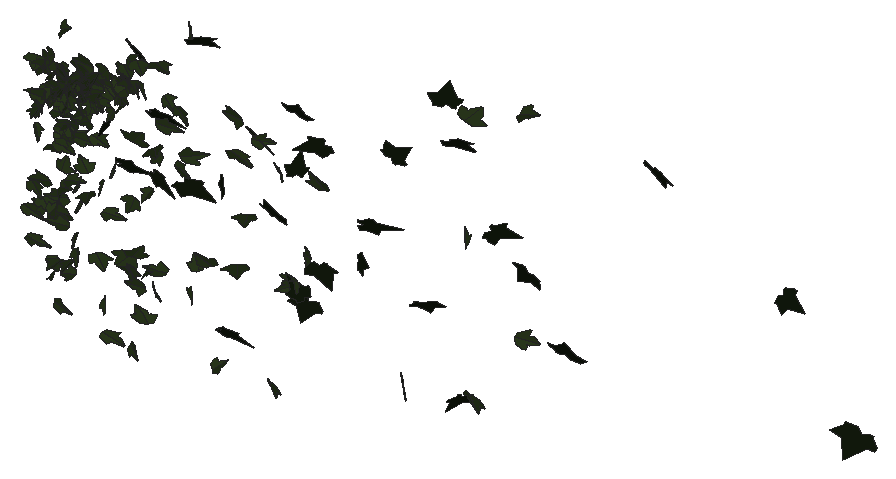
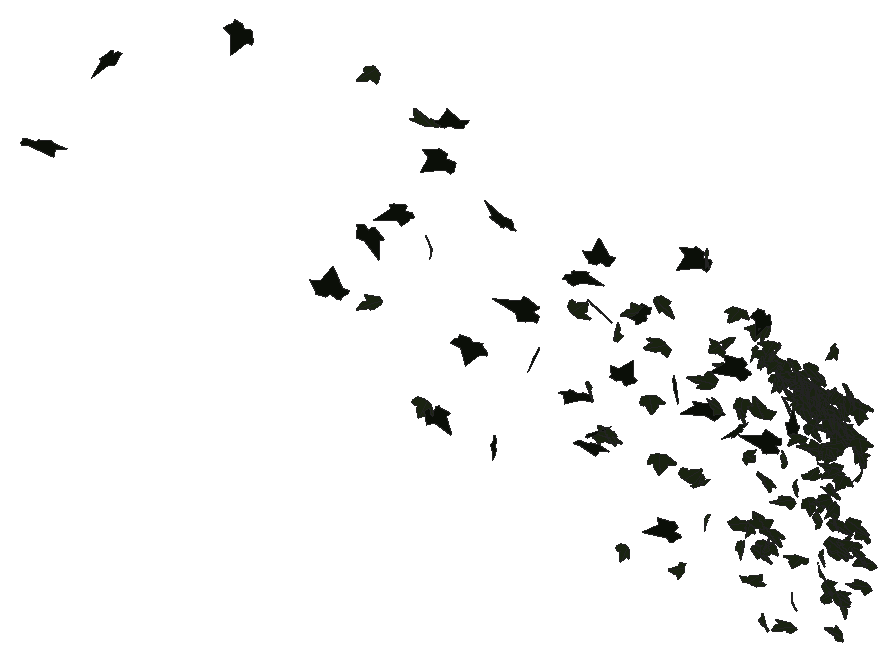
# SketchUp Ruby script. Lengths in millimetres.
U = 1.mm
M = Sketchup.active_model
def pt(a) = Geom::Point3d.new(a.map { |v| v * U })
def face(e, loops, mat)
  f = e.add_face(loops[0].map { |a| pt(a) })
  loops[1..].each { |l| e.add_face(l.map { |a| pt(a) }).erase! }
  f.material = f.back_material = mat if mat
  f
end
# faces: each face lists its corners as indices into pts; further lists are holes
def faces(e, pts, list, mat = nil) = list.each { |f| face(e, (f[0].is_a?(Array) ? f : [f]).map { |l| l.map { |i| pts[i] } }, mat) }
# xy, xz, yz: faces in a plane at the given z, y or x. An outline is a flat list of corners, or four numbers for a rectangle; further outlines are holes
def ring(l) = l.size == 4 ? [[l[0], l[1]], [l[2], l[1]], [l[2], l[3]], [l[0], l[3]]] : l.each_slice(2).to_a
def flat(e, list, mat, &to3) = list.each { |f| face(e, (f[0].is_a?(Array) ? f : [f]).map { |l| ring(l).map { |u, v| to3.(u, v) } }, mat) }
def xy(e, z, list, mat = nil) = flat(e, list, mat) { |x, y| [x, y, z] }
def xz(e, y, list, mat = nil) = flat(e, list, mat) { |x, z| [x, y, z] }
def yz(e, x, list, mat = nil) = flat(e, list, mat) { |y, z| [x, y, z] }
def lines(e, pts, list) = list.each { |a, b| e.add_line(pt(pts[a]), pt(pts[b])) }
# prism: a flat outline (further loops are holes) pulled along v
def prism(e, loops, v, mat = nil)
  f = face(e, loops, mat); d = Geom::Vector3d.new(v.map { |x| x * U })
  f.pushpull(f.normal.samedirection?(d) ? d.length : -d.length)
end
def box(e, o, s, mat = nil) = prism(e, [[o, [o[0] + s[0], o[1], o[2]], [o[0] + s[0], o[1] + s[1], o[2]], [o[0], o[1] + s[1], o[2]]]], [0, 0, s[2]], mat)
def at(x, y, z, deg = 0) = Geom::Transformation.translation(pt([x, y, z])) * Geom::Transformation.rotation(ORIGIN, Z_AXIS, deg.degrees)
def axes(o, x, y, z) = Geom::Transformation.new([*x, 0, *y, 0, *z, 0, *pt(o).to_a, 1])
def part(name) = M.definitions.add(name)
# library, detail: a bought-in or finely detailed component or shape, given as its bounding box
def library(name, o, s) = part(name).tap { |d| box(d.entities, o, s) }
def detail(e, o, s) = box(e.add_group.entities, o, s)
def put(e, d, t, mat = nil) = e.add_instance(d, t).tap { |i| i.material = mat if mat }
def group(e, t, mat = nil) = e.add_group.tap { |g| g.transformation = t; g.material = mat if mat }.entities
root = M.entities
M.materials.add("efeu1").color = [18, 25, 13]
M.materials.add("efeu2").color = [43, 57, 29]
c1 = part("ivyleaf_10")
p = [[0,12.8,-0.8],[-1.5,51.3,-10.9],[-4.9,51,-11.6],[-13.6,26.5,-7.3],[-13.2,15.9,-4.6],[-21.1,19.3,-7.2],
  [-29.5,16.3,-8.3],[-29.2,8.3,-6.2],[-19.7,-9.8,0.5],[-7.6,-13,4],[1,-12.2,5.8],[-0.4,51.1,-11.1],
  [-1.5,51.1,-10.9],[1,-12.4,5.9],[16.9,-12.4,3.5],[35.1,9.1,-5.1],[35,12.9,-6.1],[20.5,16.4,-4.9],
  [15.8,15,-3.8],[15.3,27.6,-7.1],[12.8,31.3,-7.8]]
faces(c1.entities,p,[[0,1,2,3,4,5,6,7,8,9,10],[11,12,0,13,14,15,16,17,18,19,20]],"efeu2")
c2 = part("ivyleaf_9")
p = [[39.1,54.8,31.7],[34.5,51.8,30.2],[-5.3,25.2,17.3],[-17.9,28.3,20.9],[-21.6,21.7,17],[-20.2,4.3,5.3],
  [-22.9,-0.3,2.5],[-17.1,-4,-0.6],[-2,-2.1,-1.2],[-0.7,-15.4,-10.1],[16.6,-22.3,-16.7],[21.1,-15.1,-12.5],
  [32.7,-10.7,-11],[46.1,-1.8,-6.6],[30.8,11.2,3.8]]
faces(c2.entities,p,[[0,1,2,3,4,5,6,7,8,9,10,11,12,13,14]],"efeu1")
put(root,c1,axes([1688.4,1054.2,385.2],[0.66637,0.14014,0.53567],[0.92513,0.22568,-0.37677],[-0.5046,0.59883,0.01663]))
put(root,c1,axes([1715.8,1060.3,753.9],[-0.9466,-0.39098,0.07189],[-0.06525,-0.07252,-0.63165],[0.75376,-0.49728,0.0356]))
put(root,c1,axes([1722.4,1052.4,705.3],[-0.276,-0.61082,0.15015],[-0.05742,-0.14715,-0.62778],[1.19573,-0.14805,0.00451]))
put(root,c1,axes([1727,1052.4,841.1],[-1.14001,0.22774,0.16973],[-0.33916,0.00715,-0.63849],[-0.42094,-0.62254,0.05476]))
put(root,c1,axes([1733.3,1055.6,406],[0.74106,-0.32591,-0.41907],[-0.6286,0.25817,-0.50765],[0.79103,0.51047,-0.01081]))
put(root,c1,axes([1721.7,1052.9,706.2],[0.74402,-0.51019,-0.0648],[0.0973,0.11954,-0.63278],[0.97394,0.3778,0.11272]))
put(root,c1,axes([1747.1,1057.4,489.3],[-0.51143,-0.04017,0.6118],[-1.13991,-0.12561,-0.27132],[0.24947,-0.6563,0.01448]))
put(root,c1,axes([1721.3,1049,863.4],[1.25976,0.08591,-0.01452],[-0.02826,0.00162,-0.66746],[-0.1634,0.66207,0.00352]))
put(root,c1,axes([1721,1050.8,649.2],[-0.04462,0.68269,-0.2239],[0.02754,-0.22352,-0.68306],[-1.36711,-0.02678,-0.00645]))
put(root,c1,axes([1709.9,1051.4,464.6],[0.90696,-0.15382,0.43059],[0.81416,-0.06963,-0.49831],[0.3073,0.63848,0.04939]))
put(root,c1,axes([1708.6,1045.4,301.5],[-0.4079,-0.06195,-0.61418],[1.1745,-0.03684,-0.21164],[-0.02771,-0.64945,0.07059]))
put(root,c1,axes([1742.5,1040.1,717.7],[0.01577,0.21516,-0.621],[-0.32952,0.59982,0.20552],[1.20663,0.161,0.06424]))
put(root,c1,axes([1755.7,1045.9,879.3],[0.32299,-0.47142,-0.46343],[-0.27462,0.44051,-0.50094],[1.2278,0.22254,0.00987]))
put(root,c1,axes([1723.1,1048.2,748],[0.12374,-0.0032,0.76231],[1.17016,0.45253,-0.05054],[-0.85772,0.6169,0.04103]))
put(root,c1,axes([1747.7,1052.8,758],[-0.52103,0.57291,-0.11289],[0.06869,-0.10785,-0.63481],[-1.1092,-0.27579,0.01372]))
put(root,c1,axes([1753.9,1052,750.8],[0.3947,-0.62861,-0.08831],[-0.02203,0.08915,-0.66172],[1.20791,0.20703,0.01679]))
put(root,c1,axes([1742.8,1055.4,426.1],[0.88803,0.42819,0.2143],[0.29282,0.14928,-0.63327],[-0.86298,0.49128,0.00564]))
put(root,c1,axes([1755,1048,863.6],[-1.09124,-0.35064,-0.07902],[0.18739,-0.01014,-0.66944],[0.65791,-0.5787,0.05961]))
put(root,c1,axes([1774.4,1049.3,777.5],[-0.54687,0.54467,0.20836],[-0.53322,0.07478,-0.58186],[-0.97339,-0.34697,0.20167]))
put(root,c1,axes([1774.2,1058.6,754.8],[-0.56025,-0.55661,0.109],[-0.02811,-0.11524,-0.62837],[1.07909,-0.29199,0.04022]))
put(root,c1,axes([1772.1,1059.5,774.4],[-0.28489,-0.41914,0.45869],[0.11153,-0.47923,-0.41879],[1.17728,-0.05603,0.15067]))
put(root,c1,axes([1778.9,1044.2,895.9],[0.48867,-0.47376,-0.42549],[-0.33643,0.38772,-0.53837],[1.1643,0.31088,0.02302]))
put(root,c1,axes([1775,1051.4,834],[-0.03031,-0.63857,-0.21042],[0.05202,0.20969,-0.63842],[1.27855,-0.02367,0.02099]))
put(root,c1,axes([1750.8,1057.4,778.3],[0.66661,0.03309,0.54247],[0.99021,0.16609,-0.34607],[-0.29891,0.62399,0.06335]))
put(root,c1,axes([1792.1,1056.1,398.3],[-1.02972,-0.15447,0.32085],[-0.55712,-0.13937,-0.56073],[0.3859,-0.61339,0.04661]))
put(root,c1,axes([1776.2,1058.6,775],[1.18689,-0.12873,-0.0014],[-0.00141,0.00332,-0.63677],[0.24502,0.62362,0.0031]))
put(root,c1,axes([1784.3,1047.1,222.2],[0.10096,-0.69928,-0.18249],[-0.01953,0.18224,-0.70128],[1.37531,0.05392,0.00344]))
put(root,c1,axes([1789.2,1057.7,251.6],[-0.40036,-0.48272,0.36837],[-0.23435,-0.34784,-0.52613],[1.13165,-0.24281,0.02137]))
put(root,c1,axes([1781.2,1051.9,612.5],[-0.70473,-0.48383,-0.30882],[0.34511,0.25008,-0.60922],[1.03646,-0.41224,-0.00713]))
put(root,c1,axes([1779.1,1040.1,411.1],[0.18254,0.28812,-0.61732],[0.37154,0.58564,0.30366],[1.24217,-0.21751,-0.00011]))
put(root,c1,axes([1798.2,1047.7,858.8],[-0.93446,0.33264,0.32838],[-0.53915,0.16705,-0.59279],[-0.70759,-0.56657,0.01801]))
put(root,c1,axes([1814,1059.2,407.7],[-0.56702,-0.02674,0.67681],[-1.27662,-0.091,-0.29887],[0.17897,-0.73386,0.0124]))
put(root,c1,axes([1792,1058.9,785.4],[-0.09638,-0.64206,-0.09498],[0.00722,0.09497,-0.64404],[1.23525,-0.05065,-0.00365]))
put(root,c1,axes([1766.2,1059.4,241.1],[0.2426,-0.08265,-0.6202],[1.15061,-0.14678,0.14381],[-0.30677,-0.61592,0.04895]))
put(root,c1,axes([1812.5,1050.2,462.3],[0.55085,-0.04814,-0.61462],[-1.14383,0.12923,-0.29315],[0.2614,0.66695,0.01244]))
put(root,c1,axes([1814.1,1052.4,375.5],[-0.00216,0.06306,0.64759],[-1.06342,-0.33192,0.03134],[0.63451,-0.55607,0.05473]))
put(root,c1,axes([1804.1,1057.8,795.5],[-0.30932,-0.626,0.08958],[-0.02902,-0.08858,-0.64671],[1.20318,-0.16307,0.00743]))
put(root,c1,axes([1800.8,1047.7,810],[-1.2279,-0.08263,-0.08152],[0.15996,-0.01502,-0.64995],[0.15236,-0.65013,0.02537]))
put(root,c1,axes([1804.7,1061.7,791.1],[0.06932,-0.63597,0.0421],[0.03119,-0.04122,-0.63686],[1.21263,0.03741,0.01397]))
put(root,c1,axes([1790,1051.7,721.8],[-0.35685,-0.20395,-0.57631],[0.92204,0.31807,-0.27018],[0.7096,-0.51586,0.06125]))
put(root,c1,axes([1806.8,1054.3,478.7],[0.39772,-0.63713,0.11459],[0.0925,-0.10464,-0.6704],[1.22857,0.21413,0.01338]))
put(root,c1,axes([1809.9,1047.5,792.2],[0.07675,-0.60534,-0.30444],[-0.00284,0.3049,-0.60645],[1.28957,0.0367,0.01678]))
put(root,c1,axes([1807.3,1056.1,819],[0.86009,-0.45158,-0.15955],[0.04049,0.23808,-0.61358],[0.91062,0.41594,0.17798]))
put(root,c1,axes([1794.8,1049.2,863],[1.1388,-0.14425,0.27817],[0.57836,0.12093,-0.59097],[0.14543,0.64868,0.17203]))
put(root,c1,axes([1806.5,1056.5,807.1],[0.78841,-0.50056,0.10032],[0.19872,-0.04339,-0.64765],[0.95107,0.42402,0.05216]))
put(root,c1,axes([1818.6,1062.7,780.6],[-0.60959,-0.53428,0.14995],[-0.00777,-0.17086,-0.61751],[1.0561,-0.30965,0.082]))
put(root,c1,axes([1794,1051.3,121.6],[0.06512,-0.00782,0.66223],[1.23192,-0.13988,-0.0351],[0.26664,0.64819,0.00042]))
put(root,c1,axes([1803.5,1049.7,624.5],[0.64809,0.33834,0.47524],[0.57678,0.3676,-0.47886],[-0.9487,0.45462,0.03352]))
put(root,c1,axes([1820.2,1061.9,798.4],[0.95344,0.35528,-0.1951],[-0.28637,-0.125,-0.614],[-0.71629,0.52288,-0.01422]))
put(root,c1,axes([1813.6,1050.9,552.8],[1.20898,-0.26037,-0.02043],[0.05955,0.02252,0.68574],[-0.49347,-0.63516,0.03269]))
put(root,c1,axes([1816.8,1053,753.2],[1.09075,0.28141,-0.0286],[-0.04777,-0.01377,-0.63848],[-0.53621,0.57366,-0.00129]))
put(root,c1,axes([1817.6,1046.7,868.5],[-0.34724,0.65594,0.01519],[0.02036,0.01874,-0.68067],[-1.24856,-0.18212,-0.01533]))
put(root,c1,axes([1800.1,1050.8,640.1],[0.35137,-0.03693,-0.66129],[1.11581,0.32849,0.14533],[0.58644,-0.6029,0.11969]))
put(root,c1,axes([1833.9,1055.2,695.9],[-0.89828,-0.30961,0.2979],[-0.447,-0.18464,-0.56402],[0.68473,-0.52671,0.02261]))
put(root,c1,axes([1824.3,1057.9,808.5],[1.15834,-0.1362,-0.15762],[-0.25909,0.10836,-0.61931],[0.30008,0.6193,0.0737]))
put(root,c1,axes([1822.1,1036,994.9],[-0.04137,-0.32316,-0.72112],[0.29892,0.70523,-0.32077],[1.47393,-0.1521,0.04481]))
put(root,c1,axes([1821.8,1034.8,505],[-0.13223,-0.44392,-0.63667],[0.44717,0.5972,-0.44204],[1.40788,-0.23137,0.0806]))
put(root,c1,axes([1832.6,1055.1,265.2],[-0.14744,-0.65397,0.2853],[-0.09712,-0.28116,-0.65834],[1.35444,-0.09135,-0.01615]))
put(root,c1,axes([1828.6,1042.7,754.3],[-0.0496,-0.38595,-0.51186],[0.0927,0.50961,-0.38673],[1.21654,-0.05457,0.0086]))
put(root,c1,axes([1812.7,1038.1,684.3],[0.30124,0.14682,0.65035],[0.53447,0.59156,-0.2019],[-1.15085,0.31316,0.07647]))
put(root,c1,axes([1831.9,1052.3,693.3],[-0.38434,-0.57345,-0.30825],[0.24766,0.28067,-0.6074],[1.21408,-0.23879,0.02632]))
put(root,c1,axes([1847.6,1041.2,680.7],[0.21327,0.00148,-0.71032],[-0.66242,0.62698,-0.0536],[1.17848,0.35216,0.09842]))
put(root,c1,axes([1833.3,1053.7,818.3],[-1.24449,0.00582,-0.06624],[0.12617,0.00603,-0.65389],[-0.00986,-0.65721,-0.00659]))
put(root,c1,axes([1834.9,1060.7,226.5],[-0.02377,0.25001,0.63304],[0.0662,-0.63209,0.25032],[1.29367,0.03694,-0.00118]))
put(root,c1,axes([1824.3,1050.2,777],[1.12918,0.06495,0.23202],[0.43815,0.02907,-0.59684],[-0.13525,0.63639,0.00358]))
put(root,c1,axes([1842,1054.1,810.2],[0.27755,-0.6453,0.03566],[0.02316,-0.03381,-0.66156],[1.22979,0.14627,0.00441]))
put(root,c1,axes([1848.5,1039.2,833],[-0.19813,0.25061,0.68665],[-0.45262,0.64422,-0.27118],[-1.31545,-0.25941,-0.01011]))
put(root,c1,axes([1856.7,1054.6,811.2],[-0.87759,-0.44904,0.0508],[-0.0662,-0.0371,-0.64363],[0.85752,-0.46242,0.0023]))
put(root,c1,axes([1838.1,1047.4,527],[-0.30504,-0.17347,-0.66224],[0.84208,0.49276,-0.23616],[0.99421,-0.47058,-0.00316]))
put(root,c1,axes([1829.1,1045.5,666.9],[-0.02126,-0.0111,-0.6802],[1.23412,0.20552,-0.014],[0.39148,-0.6485,0.0072]))
put(root,c1,axes([1847.5,1061.4,349.9],[0.43973,-0.48007,0.40784],[0.37948,-0.35633,-0.5324],[1.13721,0.30454,0.01996]))
put(root,c1,axes([1857.2,1053.6,835.7],[0.90322,0.44296,-0.12521],[-0.39537,0.04562,-0.626],[-0.78177,0.48869,0.17193]))
put(root,c1,axes([1872.6,1053.7,840.4],[-0.88849,-0.27826,0.38278],[-0.62834,-0.19373,-0.54347],[0.64528,-0.57178,-0.00214]))
put(root,c1,axes([1856.3,1051.6,500.4],[0.38313,-0.56917,0.33111],[-0.22355,0.30965,0.60369],[-1.23312,-0.23298,-0.00656]))
put(root,c1,axes([1861.6,1049.2,831.2],[-0.3972,-0.61594,0.02172],[-0.02366,-0.01872,-0.65031],[1.17275,-0.20899,-0.00576]))
put(root,c1,axes([1861.6,1053.7,840.9],[-0.02612,-0.66369,0.00154],[-0.00167,-0.00152,-0.66383],[1.26314,-0.01373,-0.00085]))
put(root,c1,axes([1860.2,1056.2,835.9],[-1.08161,0.31824,0.01332],[-0.01448,0.01367,-0.6513],[-0.60603,-0.5683,-0.00821]))
put(root,c1,axes([1846.5,1044.2,666.1],[0.35924,0.21563,-0.65889],[0.91786,0.44973,0.28534],[0.94787,-0.51721,-0.02659]))
put(root,c1,axes([1851.4,1057.7,302.5],[0.73888,-0.37303,0.48077],[0.63293,-0.34752,-0.53819],[0.96987,0.51097,-0.01505]))
put(root,c1,axes([1864.6,1052,804.3],[-0.81071,0.49059,-0.00356],[0.00516,-0.00236,-0.64972],[-0.93371,-0.42598,-0.0005]))
put(root,c1,axes([1866,1050.8,863.2],[0.5459,-0.60631,0.02491],[0.06173,-0.0122,-0.6703],[1.15326,0.28766,0.02409]))
put(root,c1,axes([1869.8,1052.4,855.4],[-0.61109,-0.58141,0.05639],[0.03949,-0.07566,-0.66194],[1.11103,-0.3171,0.05454]))
put(root,c1,axes([1871.3,1057,835.1],[-0.34927,-0.62046,0.05668],[-0.02412,-0.05536,-0.64702],[1.18554,-0.18392,0.00354]))
put(root,c1,axes([1870.2,1044.5,448.1],[0.50251,-0.52097,0.56106],[-0.41538,0.51764,0.58337],[-1.3967,-0.34139,0.02836]))
put(root,c1,axes([1864.9,1055.1,769],[-0.35617,0.61657,-0.03597],[0.02499,-0.03361,-0.64434],[-1.17519,-0.18758,-0.0028]))
put(root,c1,axes([1870.8,1044.2,894.5],[-1.13374,0.31932,-0.04803],[0.09865,-0.00492,-0.67559],[-0.6066,-0.59762,-0.0201]))
put(root,c1,axes([1871.5,1054.8,831],[-0.29444,-0.62445,0.09323],[0.30532,-0.13171,-0.61602],[1.16219,-0.1236,0.18545]))
put(root,c1,axes([1887.6,1054.7,747.4],[0.35703,0.28807,-0.55174],[-0.74934,-0.39139,-0.33822],[-0.91746,0.43177,0.06153]))
put(root,c1,axes([1874.3,1057,835.9],[-0.30639,0.49685,-0.39518],[0.06131,-0.40077,-0.517],[-1.20668,-0.14652,0.07407]))
put(root,c1,axes([1889.9,1053.4,857],[-1.16943,-0.01059,0.22603],[-0.42454,-0.08152,-0.61021],[0.07234,-0.64961,0.0729]))
put(root,c1,axes([1874,1057.6,835.3],[0.77443,-0.46645,0.21414],[0.30748,-0.14297,-0.61844],[0.92718,0.43702,0.02623]))
put(root,c1,axes([1898.8,1047,728.9],[-0.78024,0.13846,0.48236],[-0.92628,0.04215,-0.42575],[-0.23285,-0.63163,0.07733]))
put(root,c1,axes([1883.7,1048.7,867.1],[0.45383,-0.62034,-0.12543],[-0.01843,0.13044,-0.66356],[1.20439,0.23575,0.03711]))
put(root,c1,axes([1905.3,1042.1,909],[0.39659,-0.14312,-0.74198],[-1.04241,0.50165,-0.25058],[0.99079,0.58507,0.03336]))
put(root,c1,axes([1893.6,1049.9,578.9],[0.59202,0.64651,0.10986],[-0.10561,-0.09521,0.7174],[1.24359,-0.31586,0.00862]))
put(root,c1,axes([1896,1057.5,811.8],[-0.23273,-0.64274,-0.0049],[0.01021,0.00397,-0.65425],[1.22325,-0.12232,0.00453]))
put(root,c1,axes([1899.2,1050,500.2],[-0.52693,-0.64426,-0.03739],[0.0389,0.03191,-0.7012],[1.2276,-0.27755,0.00617]))
put(root,c1,axes([1872.2,1043.9,669.3],[0.19539,0.0143,0.67953],[1.08445,0.37283,-0.09393],[-0.70518,0.57732,0.04383]))
put(root,c1,axes([1900.3,1055.9,855.8],[-0.28634,-0.63945,-0.04545],[-0.00197,0.04693,-0.6568],[1.22006,-0.15,-0.01173]))
put(root,c1,axes([1900,1055.8,855.4],[0.27972,-0.62286,-0.15731],[-0.00532,0.16075,-0.63911],[1.22264,0.1432,0.03321]))
put(root,c1,axes([1903.5,1055.5,857.9],[-0.10457,-0.65616,-0.02433],[-0.02306,0.02543,-0.65831],[1.24946,-0.05445,-0.01419]))
put(root,c1,axes([1903.4,1057.4,834.4],[-0.09755,-0.65201,0.02266],[0.00155,-0.02279,-0.65402],[1.24166,-0.0512,0.0026]))
put(root,c1,axes([1929.9,1056.6,834.9],[-0.02841,0.03366,0.65514],[-1.09088,-0.3194,0.00335],[0.60726,-0.5722,0.03667]))
put(root,c1,axes([1908.7,1058.2,781.3],[1.23661,-0.01512,-0.06124],[-0.116,0.01261,-0.64984],[0.0309,0.65251,0.01114]))
put(root,c1,axes([1907.1,1055.6,821.6],[0.89446,0.44734,0.08411],[-0.00044,0.12113,-0.64296],[-0.8663,0.46182,0.08716]))
put(root,c1,axes([1919.4,1054.7,869.1],[0.2556,-0.64736,-0.00691],[-0.0247,0.00436,-0.66104],[1.23187,0.13441,-0.01182]))
put(root,c1,axes([1904.1,1055.1,859.3],[-0.799,-0.07668,-0.5031],[0.96657,-0.0214,-0.42054],[0.06197,-0.6549,0.07265]))
put(root,c1,axes([1918.6,1055.9,796.5],[0.19546,0.64813,-0.05276],[-0.00426,-0.05306,-0.65619],[-1.2376,0.10254,-0.00607]))
put(root,c1,axes([1930,1048.5,882],[-0.30648,-0.65598,0.03364],[0.00496,-0.03527,-0.67537],[1.25009,-0.16068,0.01093]))
put(root,c1,axes([1932.9,1049.1,820.3],[-0.43814,-0.6301,0.0833],[-0.06845,-0.07554,-0.67079],[1.2077,-0.23287,-0.0078]))
put(root,c1,axes([1907.5,1055.2,860.9],[-0.13253,0.00974,-0.65545],[1.23979,-0.07253,-0.07029],[-0.13923,-0.65513,-0.00197]))
put(root,c1,axes([1921.5,1052.1,876.3],[-1.02389,0.00696,-0.38476],[0.72478,-0.08551,-0.53402],[-0.10537,-0.65586,0.06554]))
put(root,c1,axes([1934.7,1054.9,806.4],[-0.05552,0.66023,0.00732],[-0.00029,0.00732,-0.66088],[-1.25663,-0.02917,-0.00017]))
put(root,c1,axes([1927.7,1049.9,688.4],[0.4626,0.43634,0.43011],[0.35892,0.38697,-0.49915],[-1.10945,0.30713,0.01786]))
put(root,c1,axes([1928.9,1055.7,315.1],[0.91313,0.46364,0.20836],[0.274,0.15084,-0.66715],[-0.9278,0.50085,0.00804]))
put(root,c1,axes([1934.1,1067.5,539.2],[0.34048,-0.39575,0.50296],[0.45718,-0.44254,-0.43365],[1.12898,0.29856,0.02392]))
put(root,c2,axes([1944.6,1062,710.8],[0.36289,0.37002,0.67668],[-0.57941,-0.60434,0.41624],[1.34863,-0.35921,-0.00325]))
put(root,c1,axes([1933.1,1055.2,804.8],[0.95366,-0.13334,-0.40925],[0.79009,-0.01619,0.51356],[-0.21639,-0.64677,0.07152]))
put(root,c1,axes([1959.5,1046.6,909.8],[0.90299,-0.36241,-0.31904],[-0.33246,0.28816,-0.5871],[0.85668,0.49382,0.10845]))
put(root,c1,axes([1942.9,1064.7,178.4],[0.43988,-0.26019,0.60981],[0.73998,-0.4699,-0.34786],[1.02206,0.45219,-0.0106]))
put(root,c1,axes([1956.5,1053.9,866.2],[-1.08764,0.13894,-0.30268],[0.56101,-0.06878,-0.58812],[-0.29502,-0.64302,-0.00249]))
put(root,c1,axes([1979,1053.7,783.7],[0.72244,-0.54386,-0.02655],[-0.03352,0.02009,-0.66322],[1.03576,0.37999,-0.00294]))
put(root,c1,axes([1984.1,1051.7,835.9],[0.42292,0.59015,0.22223],[-0.1428,-0.20921,0.63059],[1.19164,-0.23452,-0.00331]))
put(root,c1,axes([1985.2,1046.7,593.3],[0.43733,-0.50666,0.40543],[-0.30909,0.37151,0.55631],[-1.19569,-0.28135,0.00448]))
put(root,c1,axes([1968.4,1049.9,87.7],[0.5706,0.25988,0.56262],[0.79509,0.3769,-0.39671],[-0.87122,0.51417,0.00644]))
put(root,c1,axes([1990.6,1048.7,897],[-1.1766,0.25026,-0.0324],[0.05559,-0.01419,-0.66695],[-0.47704,-0.61891,0.00219]))
put(root,c1,axes([1974.1,1042.2,474.1],[-0.36524,-0.2351,-0.60549],[1.08079,0.24573,-0.2754],[0.60003,-0.58571,0.12749]))
put(root,c1,axes([2005.3,1052.2,844.7],[-1.15751,0.20798,0.18361],[-0.35541,0.02026,-0.64154],[-0.39048,-0.63498,0.03967]))
put(root,c1,axes([2001.7,1052.2,851.2],[0.79126,-0.50314,0.14382],[0.23327,-0.08495,-0.6515],[0.96823,0.43164,0.03942]))
put(root,c1,axes([2011.1,1043.9,938.4],[-0.36372,0.64566,0.03839],[-0.03852,0.03405,-0.67328],[-1.23039,-0.19193,0.00973]))
put(root,c1,axes([2007.7,1050.9,889.4],[0.66975,0.48528,0.30599],[0.27182,0.27356,-0.59811],[-1.05749,0.37767,0.04006]))
put(root,c1,axes([2021.7,1037.9,825.8],[-0.08116,-0.34561,-0.58866],[0.08427,0.58716,-0.34794],[1.29641,-0.0598,-0.01423]))
put(root,c1,axes([2044.7,1042.5,893.3],[0.43966,-0.04064,-0.63355],[-0.97182,0.38871,-0.21112],[0.71794,0.55105,0.1022]))
put(root,c1,axes([2038.2,1047.3,357.7],[1.34701,-0.14583,-0.30515],[-0.56036,0.08256,-0.72236],[0.31672,0.7663,0.01975]))
put(root,c1,axes([2023.9,1034.2,872.4],[0.31537,0.24204,-0.60453],[0.65084,0.49851,0.29333],[1.05469,-0.38,-0.00025]))
put(root,c1,axes([2032.5,1045.6,911.8],[-0.58475,0.59234,-0.09201],[0.10756,-0.0743,-0.6671],[-1.13579,-0.312,-0.01581]))
put(root,c1,axes([2030.6,1047.5,942.2],[0.77187,0.49376,0.23251],[0.02903,0.27931,-0.61975],[-1.03829,0.37487,0.15552]))
put(root,c1,axes([2034.7,1054.7,318.5],[-1.26975,0.22134,-0.14554],[0.24899,-0.06761,-0.70256],[-0.43838,-0.6795,0.0225]))
put(root,c1,axes([2045,1062,527.3],[1.25631,-0.36228,-0.04148],[-0.06954,0.01964,-0.75298],[0.6905,0.66112,-0.00036]))
put(root,c1,axes([2049.1,1051.7,303.5],[-0.6303,0.62006,0.1589],[0.13379,-0.14259,0.70295],[1.21087,0.33852,0.00504]))
put(root,c1,axes([2051.4,1046.5,902.8],[-0.93599,-0.46006,-0.10041],[0.23103,0.01642,-0.66977],[0.86591,-0.50167,0.07016]))
put(root,c1,axes([2052.2,1042.1,976.5],[0.12416,0.49402,0.48223],[-0.28283,0.48307,-0.47477],[-1.28308,-0.05868,0.15132]))
put(root,c2,axes([2019.2,1054.5,634.7],[0.91128,-0.16828,0.62545],[1.15802,-0.14974,-0.50609],[0.42252,0.77333,0.0381]))
put(root,c1,axes([2054.1,1060.8,890.9],[-0.55976,0.56067,-0.22412],[0.11867,-0.21976,-0.63159],[-1.14302,-0.29739,0.04419]))
put(root,c2,axes([2058.4,1046.5,1018.5],[1.17668,-0.11639,-0.51976],[-0.94931,0.15278,-0.62754],[0.35553,0.79313,0.04461]))
put(root,c1,axes([2055.8,1058.2,721.2],[-1.43496,-0.03287,0.30797],[0.58564,0.01259,0.75469],[-0.06697,0.81435,0.00077]))
put(root,c1,axes([2044.6,1058.7,71.2],[0.3596,-0.11888,0.68053],[1.03885,-0.40676,-0.22261],[0.80589,0.57738,-0.01671]))
put(root,c1,axes([2084.9,1045.1,282.9],[0.46447,-0.16605,-0.66016],[-1.02759,0.37987,-0.29515],[0.78899,0.5925,0.00422]))
put(root,c1,axes([2062.9,1049.8,370.5],[-0.85545,-0.52311,0.19366],[0.23902,0.14742,0.68969],[-1.03436,0.4667,-0.00079]))
put(root,c1,axes([2077.6,1044.4,972],[0.82125,0.50537,0.17621],[-0.01763,0.23337,-0.64661],[-1.01846,0.40347,0.15329]))
put(root,c1,axes([2088.4,1044.8,902.1],[-0.52005,0.62473,0.06912],[-0.05489,0.06282,-0.68187],[-1.19498,-0.27477,0.00124]))
put(root,c1,axes([2098.2,1051.8,181.8],[1.03318,0.39171,0.27104],[-0.42877,-0.15094,0.66937],[0.79876,-0.58769,0.00873]))
put(root,c1,axes([2102.7,1063.3,576.7],[-0.1785,-0.46555,0.51675],[0.17443,-0.52515,-0.45648],[1.31219,0.00648,0.13097]))
put(root,c1,axes([2114.6,1037.2,344.2],[-0.11954,-0.44523,-0.52849],[0.11298,0.52523,-0.44954],[1.31032,-0.08591,-0.00945]))
put(root,c1,axes([2135.3,1049,283.2],[-0.71998,0.42346,0.46618],[-0.58775,0.34922,-0.56783],[-1.04462,-0.48835,-0.00182]))
put(root,c1,axes([2134.1,1046.9,724],[-0.47886,-0.72302,-0.30589],[0.18536,0.28999,-0.76554],[1.48259,-0.26978,-0.00309]))
put(root,c1,axes([2140.1,1056.1,704.8],[0.82623,-0.52962,-0.26418],[-0.31602,0.20548,-0.68481],[1.08117,0.4648,0.00172]))
put(root,c1,axes([2149.1,1059.2,345.6],[0.25297,0.19344,0.65385],[-0.63502,-0.5625,0.23424],[1.13174,-0.35886,-0.01471]))
put(root,c2,axes([2135.2,1050.6,643.1],[0.82145,-0.65819,-0.2427],[-0.18086,0.22747,-0.78589],[1.3228,0.43983,0.04326]))
put(root,c2,axes([2130.8,1051.3,834.6],[1.47098,0.01068,0.29831],[0.56773,0.00241,-0.77297],[-0.02062,0.82846,-0.0016]))
put(root,c1,axes([2153.5,1041.6,998.8],[-0.9087,-0.39412,-0.31386],[0.46279,0.19846,-0.61911],[0.83981,-0.53581,0.00156]))
put(root,c1,axes([2180,1041.1,899.7],[0.19269,0.65541,0.20969],[0.02406,0.21014,-0.66292],[-1.30944,0.10031,0.01868]))
put(root,c1,axes([2162.2,1041.8,812.3],[-0.05894,-0.02575,0.73455],[1.25322,0.32566,0.03918],[-0.62149,0.65914,0.00934]))
put(root,c1,axes([2206.8,1060.6,689.4],[-0.1256,0.10448,-0.70337],[0.8411,-0.54737,-0.12277],[-1.06022,-0.44662,-0.01407]))
put(root,c1,axes([2211.9,1052.1,871.4],[0.94449,-0.29985,0.41047],[0.87287,0.01676,-0.54226],[0.41717,0.6438,0.20529]))
put(root,c1,axes([2263.9,1039.1,1132.9],[0.05603,-0.1645,-0.83713],[-0.27941,0.82416,-0.16711],[1.59947,0.14973,0.00013]))
put(root,c1,axes([2263.3,1041.3,311.3],[0.11125,0.15944,-0.73633],[-0.22211,0.73154,0.14914],[1.41655,0.10218,0.08121]))
put(root,c1,axes([2250,1042.1,743.9],[-0.2624,-0.247,0.79868],[0.67128,0.71671,0.28254],[-1.44253,0.37845,-0.0138]))
put(root,c2,axes([2249.8,1039.1,661.3],[0.08876,-0.22895,-0.81104],[0.68163,0.74066,-0.18849],[1.45185,-0.33374,0.13808]))
put(root,c1,axes([2286.8,1041.7,414.6],[0.36465,0.71191,-0.07057],[0.0336,0.06833,0.73724],[1.36113,-0.19241,0.00071]))
put(root,c2,axes([2280.4,1039.7,1119.5],[1.2089,0.4711,0.32823],[0.49811,0.1981,-0.79082],[-0.97263,0.68699,0.00296]))
put(root,c1,axes([2316.9,1052.2,430.9],[-0.95227,-0.20557,-0.47401],[-0.82278,-0.19476,0.54081],[-0.53847,0.66114,0.01192]))
put(root,c1,axes([2351.3,1038,128.4],[0.07055,0.12736,-0.75036],[0.56023,0.69039,0.13172],[1.33578,-0.29627,-0.01561]))
put(root,c2,axes([2376.5,1038.9,700.5],[0.08881,0.02468,-0.80853],[-1.36228,0.37851,-0.02976],[0.71712,0.71598,0.0436]))
put(root,c2,axes([2371.9,1049.2,242.5],[1.32805,-0.08585,0.31372],[0.5895,-0.05121,-0.70296],[0.18889,0.76336,-0.01187]))
put(root,c1,axes([2427.2,1037.1,929.9],[0.57068,-0.10603,-0.82326],[-1.0577,0.62454,-0.28285],[1.17344,0.61451,0.14543]))
put(root,c1,axes([2416.5,1052.4,455.3],[-1.00082,-0.67296,-0.06046],[0.06977,0.04808,-0.85405],[1.28404,-0.52714,-0.00071]))
put(root,c1,axes([2410.2,1050.8,807.1],[-1.03306,0.05706,-0.5071],[0.96036,-0.05025,-0.54579],[-0.14465,-0.74112,-0.00204]))
put(root,c1,axes([2450.6,1050.9,624.6],[-0.86311,-0.59208,0.02958],[-0.02797,-0.02601,-0.74579],[1.12791,-0.45372,0.00415]))
put(root,c2,axes([2461.5,1061.2,886.8],[0.91747,-0.59856,0.20369],[0.26696,-0.14851,-0.76839],[1.17334,0.50182,0.01555]))
put(root,c1,axes([2492.5,1043.5,879.9],[0.20673,0.11928,0.73924],[0.47321,0.69886,-0.1493],[-1.34427,0.26435,0.06113]))
put(root,c1,axes([2535.2,1054.1,131],[-1.0519,0.51618,0.04112],[-0.06156,0.0256,-0.75624],[-0.98358,-0.55364,0.00336]))
put(root,c2,axes([2542.4,1056.3,659.1],[1.00878,-0.48981,0.33141],[-0.44505,0.23519,0.72159],[-1.03381,-0.5792,0.01275]))
put(root,c1,axes([2555.7,1064.8,786.7],[-0.83146,0.49632,0.37938],[0.44393,-0.29987,0.6609],[1.10296,0.49484,0.01999]))
put(root,c1,axes([2609.6,1059.3,461.3],[0.5581,0.25277,-0.66649],[-1.08711,-0.34779,-0.38322],[-0.81155,0.63972,0.055]))
put(root,c1,axes([2606.1,1054.1,476.8],[1.10602,-0.3353,-0.37151],[-0.57725,0.21687,-0.67018],[0.75758,0.65476,0.03173]))
put(root,c2,axes([2614.3,1059.2,1001.5],[1.38298,-0.22595,0.13053],[-0.21291,0.07917,0.75983],[-0.44868,-0.73403,0.04177]))
put(root,c2,axes([2632.7,1041,830.8],[-1.14195,0.53112,-0.11047],[-0.15965,0.0719,0.80131],[1.02004,0.60585,0.00175]))
put(root,c2,axes([2641.9,1053.9,446.4],[-0.90569,-0.57984,0.17724],[0.2153,0.13644,0.75012],[-1.13369,0.48914,0.00086]))
put(root,c2,axes([2652.9,1066.6,422],[-1.18689,-0.41385,-0.21587],[0.34125,0.12022,-0.74846],[0.8202,-0.64889,-0.00098]))
put(root,c1,axes([2672.2,1041.2,582],[0.2537,-0.34067,-0.68513],[-0.4757,0.63791,-0.36582],[1.37636,0.28327,-0.00015]))
put(root,c2,axes([2700.5,1065.6,928.9],[-0.0921,-0.12472,-0.7707],[-0.4543,-0.73284,0.13358],[-1.41472,0.24345,0.00728]))
put(root,c1,axes([2708.7,1050.3,809.3],[-1.24469,0.22592,-0.36703],[-0.67556,0.09597,0.69156],[0.46522,0.74379,0.02225]))
put(root,c2,axes([2701.5,1054.3,555.2],[-0.52811,-0.53271,-0.5056],[0.50004,0.43271,-0.60011],[1.30529,-0.3813,0.02533]))
put(root,c2,axes([2847.8,1043.9,628.2],[0.46556,-0.08673,-0.76267],[-1.01698,0.55541,-0.23455],[1.04876,0.57709,0.11112]))
put(root,c2,axes([2868.2,1042.8,750],[0.83017,0.45354,-0.61978],[0.69878,0.50289,0.62641],[1.2838,-0.56701,0.05982]))
put(root,c2,axes([2958.3,1048.9,990.4],[-0.51904,0.3486,0.68757],[0.85362,-0.52142,0.44227],[1.19327,0.52464,-0.01731]))
put(root,c2,axes([2976.8,1065.4,301.1],[-0.04534,0.00622,-0.82368],[1.3621,-0.40778,-0.02378],[-0.77608,-0.71606,0.00638]))
put(root,c2,axes([3072.3,1044.5,576.6],[0.96823,0.6559,-0.09298],[-0.12987,-0.06472,-0.82995],[-1.25408,0.5131,0.01417]))
put(root,c2,axes([3150.6,1041.6,1228.6],[-1.12421,-0.2827,0.53435],[1.01305,0.11091,0.6471],[-0.54538,0.78876,0.10053]))
put(root,c2,axes([3194.5,1052.1,324.1],[-0.14696,0.63035,-0.56912],[0.17289,-0.56206,-0.63485],[-1.60703,-0.11811,-0.01626]))
put(root,c2,axes([3168.6,1041.4,1114.2],[1.32776,0.41356,0.2375],[0.38622,0.12341,-0.81101],[-0.82138,0.72656,0.00257]))
put(root,c1,axes([3221.4,1040.3,818.4],[0.54507,-0.37503,0.75007],[-0.92937,0.56978,0.47134],[-1.29752,-0.56566,-0.02251]))
put(root,c1,axes([3233.4,1051.3,336.2],[-1.41959,0.42304,-0.01831],[0.03031,-0.00904,-0.85751],[-0.80531,-0.74607,0.00001]))
put(root,c1,axes([3226.6,1042.9,1207.8],[1.44241,-0.00167,-0.39053],[0.73943,0.08979,0.75359],[0.07546,-0.84785,0.08058]))
put(root,c2,axes([3321.3,1030.2,894.1],[0.26139,0.14282,-0.8781],[-0.07102,0.88864,0.1387],[1.69166,0.01524,0.1415]))
put(root,c2,axes([3431.7,1042.7,798.9],[0.86336,0.06676,-0.79201],[-1.49596,-0.09761,-0.45843],[-0.22441,0.90749,0.00896]))
put(root,c1,axes([3409.7,1041.1,587.2],[0.16283,0.35048,0.7985],[0.35354,0.7766,-0.36077],[-1.62157,0.20451,0.00153]))
put(root,c1,axes([3423.7,1035.8,1295.5],[-0.38002,-0.32645,-0.7891],[0.7507,0.6835,-0.38257],[1.44149,-0.44201,-0.00879]))
put(root,c2,axes([3548,1063.3,576.3],[1.59809,-0.32422,0.23219],[-0.41158,0.08454,0.90011],[-0.63768,-0.86709,0.00094]))
put(root,c2,axes([3865.4,1046.4,1271.6],[1.59767,-0.08773,-0.5078],[-0.95631,0.07603,-0.8438],[0.21763,0.97815,0.02004]))
put(root,c2,axes([4320.1,1046.1,1035.2],[0.40701,-0.40455,-0.93147],[-0.72898,0.84947,-0.45687],[1.79001,0.43793,0.02574]))
put(root,c2,axes([4567.4,1061.7,685.3],[-1.60579,-0.64162,-0.07423],[0.1174,0.04151,-1.05997],[1.22366,-0.84597,0.00429]))
